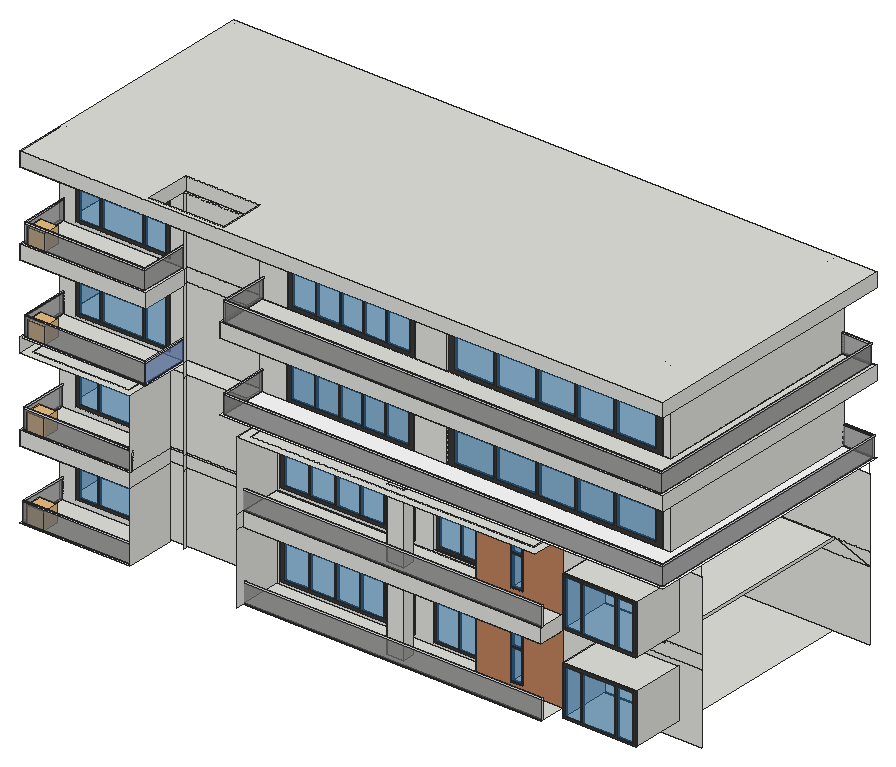
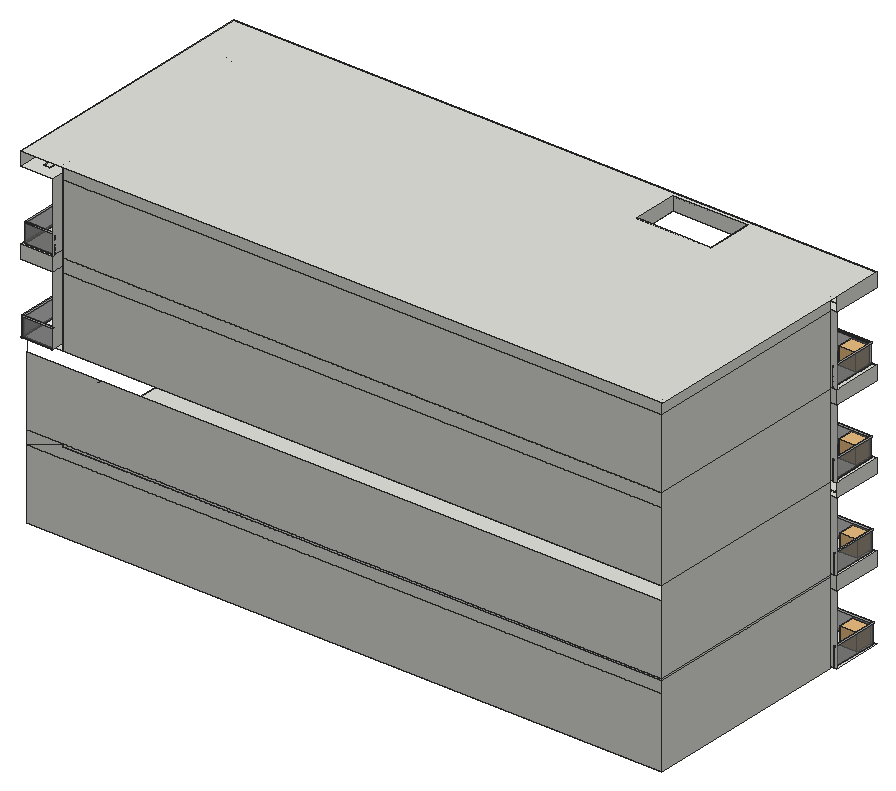
# SketchUp Ruby script. Lengths in inches.
U = 1.inch
M = Sketchup.active_model
def pt(a) = Geom::Point3d.new(a.map { |v| v * U })
def face(e, loops, mat)
  f = e.add_face(loops[0].map { |a| pt(a) })
  loops[1..].each { |l| e.add_face(l.map { |a| pt(a) }).erase! }
  f.material = f.back_material = mat if mat
  f
end
# faces: each face lists its corners as indices into pts; further lists are holes
def faces(e, pts, list, mat = nil) = list.each { |f| face(e, (f[0].is_a?(Array) ? f : [f]).map { |l| l.map { |i| pts[i] } }, mat) }
# xy, xz, yz: faces in a plane at the given z, y or x. An outline is a flat list of corners, or four numbers for a rectangle; further outlines are holes
def ring(l) = l.size == 4 ? [[l[0], l[1]], [l[2], l[1]], [l[2], l[3]], [l[0], l[3]]] : l.each_slice(2).to_a
def flat(e, list, mat, &to3) = list.each { |f| face(e, (f[0].is_a?(Array) ? f : [f]).map { |l| ring(l).map { |u, v| to3.(u, v) } }, mat) }
def xy(e, z, list, mat = nil) = flat(e, list, mat) { |x, y| [x, y, z] }
def xz(e, y, list, mat = nil) = flat(e, list, mat) { |x, z| [x, y, z] }
def yz(e, x, list, mat = nil) = flat(e, list, mat) { |y, z| [x, y, z] }
def lines(e, pts, list) = list.each { |a, b| e.add_line(pt(pts[a]), pt(pts[b])) }
# prism: a flat outline (further loops are holes) pulled along v
def prism(e, loops, v, mat = nil)
  f = face(e, loops, mat); d = Geom::Vector3d.new(v.map { |x| x * U })
  f.pushpull(f.normal.samedirection?(d) ? d.length : -d.length)
end
def box(e, o, s, mat = nil) = prism(e, [[o, [o[0] + s[0], o[1], o[2]], [o[0] + s[0], o[1] + s[1], o[2]], [o[0], o[1] + s[1], o[2]]]], [0, 0, s[2]], mat)
def at(x, y, z, deg = 0) = Geom::Transformation.translation(pt([x, y, z])) * Geom::Transformation.rotation(ORIGIN, Z_AXIS, deg.degrees)
def axes(o, x, y, z) = Geom::Transformation.new([*x, 0, *y, 0, *z, 0, *pt(o).to_a, 1])
def part(name) = M.definitions.add(name)
# library, detail: a bought-in or finely detailed component or shape, given as its bounding box
def library(name, o, s) = part(name).tap { |d| box(d.entities, o, s) }
def detail(e, o, s) = box(e.add_group.entities, o, s)
def put(e, d, t, mat = nil) = e.add_instance(d, t).tap { |i| i.material = mat if mat }
def group(e, t, mat = nil) = e.add_group.tap { |g| g.transformation = t; g.material = mat if mat }.entities
root = M.entities
M.materials.add("[Color M00]").color = [255, 255, 255]
M.materials.add("[Color M07]").color = [58, 58, 58]
M.materials.add("[Metal Silver]").color = [234, 233, 238]
M.materials.add("[Translucent Glass Blue]").color = [100, 149, 237]
M.materials["[Translucent Glass Blue]"].alpha = 0.5
M.materials.add("[Translucent Glass Gray]").color = [40, 128, 199]
M.materials["[Translucent Glass Gray]"].alpha = 0.5
M.materials.add("[Translucent Glass Gray]1").color = [128, 128, 128]
M.materials["[Translucent Glass Gray]1"].alpha = 0.5
M.materials.add("[Wood Veneer 02]").color = [190, 128, 91]
c1 = library("plants",[-16.3,-15.81,0],[32.6,31.62,37.8])
c2 = part("Group\#3")
xy(c2.entities,0,[[0,0,103.1875,6]],"[Color M07]")
xy(c2.entities,6.75,[[6.75,0,49.1,6],[51.71,0,96.4375,6]],"[Color M07]")
xy(c2.entities,160.21,[[6.75,0,49.1,6],[51.71,0,96.4375,6]],"[Color M07]")
xy(c2.entities,166.96,[[0,0,103.1875,6]],"[Color M07]")
xz(c2.entities,0,[[[0,0,103.1875,166.96],[51.71,6.75,96.4375,160.21],[6.75,6.75,49.1,160.21]]],"[Color M07]")
xz(c2.entities,0,[[6.75,6.75,49.1,160.21],[51.71,6.75,96.4375,160.21]],"[Translucent Glass Gray]")
xz(c2.entities,6,[[[0,0,103.1875,166.96],[51.71,6.75,96.4375,160.21],[6.75,6.75,49.1,160.21]]],"[Color M07]")
yz(c2.entities,0,[[0,0,6,166.96]],"[Color M07]")
yz(c2.entities,6.75,[[0,6.75,6,160.21]],"[Color M07]")
yz(c2.entities,49.1,[[0,6.75,6,160.21]],"[Color M07]")
yz(c2.entities,51.71,[[0,6.75,6,160.21]],"[Color M07]")
yz(c2.entities,96.4375,[[0,6.75,6,160.21]],"[Color M07]")
yz(c2.entities,103.1875,[[0,0,6,166.96]],"[Color M07]")
c3 = part("Group\#2")
xy(c3.entities,0,[[0,0,266.875,6]],"[Color M07]")
xy(c3.entities,9.27,[[9.27,0,57.67,6],[61.37,0,109.48,6],[113.18,0,157.6,6],[161.3,0,205.85,6],[209.55,0,257.6,6]],"[Color M07]")
xy(c3.entities,155.66,[[9.27,0,57.67,6],[61.37,0,109.48,6],[113.18,0,157.6,6],[161.3,0,205.85,6],[209.55,0,257.6,6]],"[Color M07]")
xy(c3.entities,164.9375,[[0,0,266.875,6]],"[Color M07]")
xz(c3.entities,0,[[[0,0,266.875,164.9375],[9.27,9.27,57.67,155.66],[61.37,9.27,109.48,155.66],[209.55,9.27,257.6,155.66],[161.3,9.27,205.85,155.66],[113.18,9.27,157.6,155.66]]],"[Color M07]")
xz(c3.entities,0,[[9.27,9.27,57.67,155.66],[61.37,9.27,109.48,155.66],[113.18,9.27,157.6,155.66],[161.3,9.27,205.85,155.66],[209.55,9.27,257.6,155.66]],"[Translucent Glass Gray]")
xz(c3.entities,6,[[[0,0,266.875,164.9375],[9.27,9.27,57.67,155.66],[61.37,9.27,109.48,155.66],[209.55,9.27,257.6,155.66],[161.3,9.27,205.85,155.66],[113.18,9.27,157.6,155.66]]],"[Color M07]")
yz(c3.entities,0,[[0,0,6,164.9375]],"[Color M07]")
yz(c3.entities,9.27,[[0,9.27,6,155.66]],"[Color M07]")
yz(c3.entities,57.67,[[0,9.27,6,155.66]],"[Color M07]")
yz(c3.entities,61.37,[[0,9.27,6,155.66]],"[Color M07]")
yz(c3.entities,109.48,[[0,9.27,6,155.66]],"[Color M07]")
yz(c3.entities,113.18,[[0,9.27,6,155.66]],"[Color M07]")
yz(c3.entities,157.6,[[0,9.27,6,155.66]],"[Color M07]")
yz(c3.entities,161.3,[[0,9.27,6,155.66]],"[Color M07]")
yz(c3.entities,205.85,[[0,9.27,6,155.66]],"[Color M07]")
yz(c3.entities,209.55,[[0,9.27,6,155.66]],"[Color M07]")
yz(c3.entities,257.6,[[0,9.27,6,155.66]],"[Color M07]")
yz(c3.entities,266.875,[[0,0,6,164.9375]],"[Color M07]")
c4 = part("Group\#4")
xy(c4.entities,0,[[0,0,117.92,3.42]],"[Color M07]")
xy(c4.entities,5.06,[[5.06,0,29.89,3.42],[33.27,0,84.5,3.42],[87.88,0,112.86,3.42]],"[Color M07]")
xy(c4.entities,112.86,[[5.06,0,29.89,3.42],[33.27,0,84.5,3.42],[87.88,0,112.86,3.42]],"[Color M07]")
xy(c4.entities,117.92,[[0,0,117.92,3.42]],"[Color M07]")
xz(c4.entities,0,[[[0,0,117.92,117.92],[33.27,5.06,84.5,112.86],[87.88,5.06,112.86,112.86],[5.06,5.06,29.89,112.86]]],"[Color M07]")
xz(c4.entities,0,[[5.06,5.06,29.89,112.86],[33.27,5.06,84.5,112.86],[87.88,5.06,112.86,112.86]],"[Translucent Glass Gray]")
xz(c4.entities,3.42,[[[0,0,117.92,117.92],[33.27,5.06,84.5,112.86],[87.88,5.06,112.86,112.86],[5.06,5.06,29.89,112.86]]],"[Color M07]")
yz(c4.entities,0,[[0,0,3.42,117.92]],"[Color M07]")
yz(c4.entities,5.06,[[0,5.06,3.42,112.86]],"[Color M07]")
yz(c4.entities,29.89,[[0,5.06,3.42,112.86]],"[Color M07]")
yz(c4.entities,33.27,[[0,5.06,3.42,112.86]],"[Color M07]")
yz(c4.entities,84.5,[[0,5.06,3.42,112.86]],"[Color M07]")
yz(c4.entities,87.88,[[0,5.06,3.42,112.86]],"[Color M07]")
yz(c4.entities,112.86,[[0,5.06,3.42,112.86]],"[Color M07]")
yz(c4.entities,117.92,[[0,0,3.42,117.92]],"[Color M07]")
c5 = part("Group\#5")
xy(c5.entities,0,[[0,0,33.625,2.4375]],"[Color M07]")
xy(c5.entities,2.77,[[2.77,0,30.85,2.4375]],"[Color M07]")
xy(c5.entities,92.73,[[2.77,0,30.85,2.4375]],"[Color M07]")
xy(c5.entities,95.66,[[2.77,0,30.85,2.4375]],"[Color M07]")
xy(c5.entities,164.1,[[2.77,0,30.85,2.4375]],"[Color M07]")
xy(c5.entities,166.875,[[0,0,33.625,2.4375]],"[Color M07]")
xz(c5.entities,0,[[[0,0,33.625,166.875],[2.77,2.77,30.85,92.73],[2.77,95.66,30.85,164.1]]],"[Color M07]")
xz(c5.entities,0,[[2.77,2.77,30.85,92.73],[2.77,95.66,30.85,164.1]],"[Translucent Glass Gray]")
xz(c5.entities,2.4375,[[[0,0,33.625,166.875],[2.77,2.77,30.85,92.73],[2.77,95.66,30.85,164.1]]],"[Color M07]")
yz(c5.entities,0,[[0,0,2.4375,166.875]],"[Color M07]")
yz(c5.entities,2.77,[[0,2.77,2.4375,92.73],[0,95.66,2.4375,164.1]],"[Color M07]")
yz(c5.entities,30.85,[[0,2.77,2.4375,92.73],[0,95.66,2.4375,164.1]],"[Color M07]")
yz(c5.entities,33.625,[[0,0,2.4375,166.875]],"[Color M07]")
xy(root,585,[[0,191.16,284.54,191.16,284.54,195.23,3.5,195.23,3.5,320.73,0,320.73],[3.5,195.23,3.5,320.73,5.5,320.73,5.5,197.23,284.54,197.23,284.54,195.23],[5.5,197.23,284.54,320.73],[559.99,210.66,1334.26,213.98],[559.99,213.98,1334.26,215.98],
  [[559.99,215.98,1334.26,215.98,1334.26,280.1,1109.39,280.1,1109.39,320.73,559.99,320.73],[917.6,232.38,960.55,263.125]],[917.6,232.38,960.55,263.125],[1109.39,280.1,1334.26,320.73],[9.75,328.54,1561.7,873.45]])
xy(root,589.69,[[967.92,320.73,1101.04,328.54]])
xy(root,590.74,[[568.97,320.73,917.6,328.54]])
xy(root,596.29,[[40.45,320.73,260.7,328.54]])
xy(root,599.96,[[1200.375,280.1,1230.875,328.54]])
xy(root,625.17,[[1405.04,191.16,1595.91,328.54]])
xy(root,633,[[3.5,195.23,3.5,320.73,5.5,320.73,5.5,197.23,284.54,197.23,284.54,195.23],[559.99,213.98,1334.26,215.98]],"[Metal Silver]")
xy(root,637,[[3.5,195.23,284.54,195.23,284.54,197.23,5.5,197.23,5.5,320.73,3.5,320.73],[559.99,213.98,1334.26,215.98]],"[Metal Silver]")
xy(root,733.42,[[568.97,320.73,917.6,328.54],[967.92,320.73,1101.04,328.54]])
xy(root,746.15,[[1200.375,280.1,1230.875,328.54]])
xy(root,750.17,[[40.45,320.73,260.7,328.54]])
xy(root,753.48,[[1405.04,191.16,1595.91,328.54]])
xy(root,757,[[[578.25,228.93,578.25,302.47,1091.125,302.47,1091.125,261.84,1316,261.84,1316,228.93],[917.6,232.38,960.55,263.125]]])
xy(root,760,[[20.05,211.22,264.48,300.67]])
xy(root,765,[[[0,191.16,284.54,320.73],[20.05,211.22,264.48,300.67]],[[559.99,210.66,559.99,320.73,1109.39,320.73,1109.39,280.1,1334.26,280.1,1334.26,210.66],[578.25,228.93,1316,228.93,1316,261.84,1091.125,261.84,1091.125,302.47,578.25,302.47]],[20.05,211.22,264.48,300.67],[[578.25,228.93,1316,228.93,1316,261.84,1091.125,261.84,1091.125,302.47,578.25,302.47],[917.6,232.38,960.55,263.125]],[917.6,232.38,960.55,263.125],
  [1109.39,280.1,1334.26,320.73]])
xy(root,795,[[9.75,328.54,1561.7,873.45]])
xy(root,801,[[0,191.16,284.54,191.16,284.54,196.41,4.5,196.41,4.5,320.73,0,320.73],[4.5,196.41,4.5,320.73,6.5,320.73,6.5,198.41,284.54,198.41,284.54,196.41],[6.5,198.41,284.54,320.73],[559.99,210.66,1334.26,213.16],[559.99,213.16,1334.26,215.16],
  [[559.99,215.16,1334.26,215.16,1334.26,280.1,1109.39,280.1,1109.39,320.73,559.99,320.73],[917.6,232.38,960.55,263.125]],[917.6,232.38,960.55,263.125],[1109.39,280.1,1334.26,320.73],[9.75,328.54,1561.7,873.45]])
xy(root,805.07,[[967.92,320.73,1101.04,328.54]])
xy(root,808.99,[[568.97,320.73,917.6,328.54]])
xy(root,812.92,[[40.45,320.73,260.7,328.54]])
xy(root,818.15,[[1200.375,280.1,1230.875,328.54]])
xy(root,832.73,[[1405.04,191.16,1595.91,328.54]])
xy(root,849,[[4.5,196.41,4.5,320.73,6.5,320.73,6.5,198.41,284.54,198.41,284.54,196.41],[559.99,213.16,1334.26,215.16]],"[Metal Silver]")
xy(root,853,[[4.5,196.41,284.54,196.41,284.54,198.41,6.5,198.41,6.5,320.73,4.5,320.73],[559.99,213.16,1334.26,215.16]],"[Metal Silver]")
xy(root,958.6,[[568.97,320.73,917.6,328.54],[967.92,320.73,1101.04,328.54]])
xy(root,961.04,[[1405.04,191.16,1595.91,328.54]])
xy(root,964.33,[[1200.375,280.1,1230.875,328.54]])
xy(root,966.79,[[40.45,320.73,260.7,328.54]])
xy(root,973,[[[581.03,212.21,581.03,299.68,1088.34,299.68,1088.34,259.06,1313.21,259.06,1313.21,212.21],[917.6,232.38,960.55,263.125]]])
xy(root,976,[[17.39,208.55,267.15,303.34]])
xy(root,981,[[[0,191.16,284.54,320.73],[17.39,208.55,267.15,303.34]],[[559.99,191.16,559.99,320.73,1109.39,320.73,1109.39,280.1,1334.26,280.1,1334.26,191.16],[581.03,212.21,1313.21,212.21,1313.21,259.06,1088.34,259.06,1088.34,299.68,581.03,299.68]],[17.39,208.55,267.15,303.34],[[581.03,212.21,1313.21,212.21,1313.21,259.06,1088.34,259.06,1088.34,299.68,581.03,299.68],[917.6,232.38,960.55,263.125]],[917.6,232.38,960.55,263.125]])
xy(root,1017,[[0,191.16,324.77,191.16,324.77,320.73,320.15,320.73,320.15,196.41,6.6875,196.41,6.6875,320.73,0,320.73],[6.6875,196.41,6.6875,320.73,8.6875,320.73,8.6875,198.41,318.15,198.41,318.15,320.73,320.15,320.73,320.15,196.41],[8.6875,198.41,318.15,320.73],[587.47,320.73,915.35,328.54],[915.35,320.73,1002.83,328.54],
  [1002.83,320.73,1561.7,328.54],[1561.7,320.73,1581.35,328.54],[9.75,328.54,1561.7,873.45],[1561.7,328.54,1581.35,873.45]])
xy(root,1017,[[518.01,191.16,518.01,320.73,523.33,320.73,523.33,196.23,1661.42,196.23,1661.42,882.43,1665.48,882.45,1665.48,191.16],[525.33,198.23,525.33,320.73,1581.35,320.73,1581.35,879.63,1659.42,879.63,1659.42,198.23],[1581.35,879.63,1581.35,881.99,1659.42,882.42,1659.42,879.63],[1581.35,881.99,1659.42,882.42,1659.42,882.45,1581.35,882.45],[1659.42,882.42,1661.42,882.43,1661.42,882.45,1659.42,882.45],
  [1661.42,882.43,1665.48,882.45,1661.42,882.45]],"[Color M00]")
xy(root,1017,[[523.33,196.23,523.33,320.73,525.33,320.73,525.33,198.23,1659.42,198.23,1659.42,882.42,1661.42,882.43,1661.42,196.23]],"[Translucent Glass Gray]1")
xy(root,1024.1,[[41.07,320.73,283.01,328.54]])
xy(root,1065,[[523.33,196.23,523.33,320.73,525.33,320.73,525.33,198.23,1659.42,198.23,1659.42,882.42,1661.42,882.43,1661.42,196.23],[6.6875,196.41,6.6875,320.73,8.6875,320.73,8.6875,198.41,318.15,198.41,318.15,320.73,320.15,320.73,320.15,196.41],[1581.35,879.63,1581.35,881.99,1659.42,882.42,1659.42,879.63]],"[Metal Silver]")
xy(root,1069,[[523.33,196.23,1661.42,196.23,1661.42,882.43,1581.35,881.99,1581.35,879.63,1659.42,879.63,1659.42,198.23,525.33,198.23,525.33,320.73,523.33,320.73],[6.6875,196.41,320.15,196.41,320.15,320.73,318.15,320.73,318.15,198.41,8.6875,198.41,8.6875,320.73,6.6875,320.73]],"[Metal Silver]")
xy(root,1160.71,[[587.47,320.73,915.35,328.54],[1002.83,320.73,1561.7,328.54]])
xy(root,1187.47,[[41.07,320.73,283.01,328.54]])
xy(root,1189,[[552.125,216.56,552.125,295.33,1606.75,295.33,1606.75,857.05,1640.08,857.05,1640.08,216.56]])
xy(root,1197,[[[0,191.16,324.77,320.73],[20.91,212.07,303.87,299.82]],[[518.01,191.16,518.01,320.73,1581.35,320.73,1581.35,882.45,1665.48,882.45,1665.48,191.16],[552.125,216.56,1640.08,216.56,1640.08,857.05,1606.75,857.05,1606.75,295.33,552.125,295.33]],[20.91,212.07,303.87,299.82],[552.125,216.56,1640.08,216.56,1640.08,857.05,1606.75,857.05,1606.75,295.33,552.125,295.33]])
xy(root,1233,[[0,191.16,324.77,191.16,324.77,320.73,319.34,320.73,319.34,196.04,8.125,196.04,8.125,320.73,0,320.73],[518.01,191.16,1665.48,191.16,1665.48,882.45,1581.35,882.45,1581.35,877.14,1658.85,877.14,1658.85,195.23,524.95,195.23,524.95,320.73,518.01,320.73],[524.95,195.23,524.95,320.73,526.95,320.73,526.95,197.23,1656.85,197.23,1656.85,875.14,1658.85,875.14,1658.85,195.23],[8.125,196.04,8.125,320.73,10.125,320.73,10.125,198.04,317.34,198.04,317.34,320.73,319.34,320.73,319.34,196.04],[526.95,197.23,1656.85,197.23,1656.85,875.14,1581.35,875.14,1581.35,320.73,526.95,320.73],
  [10.125,198.04,317.34,320.73],[590.16,320.73,918.03,328.54],[1002.83,320.73,1561.7,328.54],[9.75,328.54,1561.7,873.45]])
xy(root,1241.47,[[41.07,320.73,283.01,328.54]])
xy(root,1281,[[524.95,195.23,524.95,320.73,526.95,320.73,526.95,197.23,1656.85,197.23,1656.85,875.14,1658.85,875.14,1658.85,195.23],[8.125,196.04,8.125,320.73,10.125,320.73,10.125,198.04,317.34,198.04,317.34,320.73,319.34,320.73,319.34,196.04],[1581.35,875.14,1658.85,877.14]],"[Metal Silver]")
xy(root,1285,[[524.95,195.23,1658.85,195.23,1658.85,877.14,1581.35,877.14,1581.35,875.14,1656.85,875.14,1656.85,197.23,526.95,197.23,526.95,320.73,524.95,320.73],[8.125,196.04,319.34,196.04,319.34,320.73,317.34,320.73,317.34,198.04,10.125,198.04,10.125,320.73,8.125,320.73]],"[Metal Silver]")
xy(root,1383.58,[[590.16,320.73,918.03,328.54],[1002.83,320.73,1561.7,328.54]])
xy(root,1404.85,[[41.07,320.73,283.01,328.54]])
xy(root,1405,[[24.96,217.75,297.46,291.5625],[552.125,225.28,552.125,286.62,1615.47,286.62,1615.47,848.34,1631.37,848.34,1631.37,225.28]])
xy(root,1413,[[[0,191.16,0,320.73,324.77,320.73,324.77,202.74,518.01,202.74,518.01,191.16],[24.96,217.75,297.46,291.5625]],[[518.01,191.16,518.01,320.73,1581.35,320.73,1581.35,882.45,1665.48,882.45,1665.48,191.16],[552.125,225.28,1631.37,225.28,1631.37,848.34,1615.47,848.34,1615.47,286.62,552.125,286.62]],[24.96,217.75,297.46,291.5625],[552.125,225.28,1631.37,225.28,1631.37,848.34,1615.47,848.34,1615.47,286.62,552.125,286.62],[324.77,313.48,334,320.73],
  [341.5,313.48,349,320.73],[356.5,313.48,364,320.73],[371.5,313.48,379,320.73],[386.5,313.48,394,320.73],[401.5,313.48,409,320.73],
  [416.5,313.48,424,320.73],[431.5,313.48,439,320.73],[446.5,313.48,454,320.73],[461.5,313.48,469,320.73],[476.5,313.48,484,320.73],
  [491.5,313.48,499,320.73],[506.5,313.48,514,320.73]])
xy(root,1443,[[9.75,328.54,1561.7,873.45]])
xy(root,1449,[[[0,191.16,1665.48,882.45],[324.77,202.74,518.01,320.73]]])
xz(root,191.16,[[0,765,284.54,801],[0,1197,324.77,1233],[518.01,1197,1665.48,1233],[0,1413,1665.48,1449]])
xz(root,195.23,[[3.5,633,284.54,637],[524.95,1281,1658.85,1285]],"[Metal Silver]")
xz(root,195.23,[[3.5,585,284.54,633],[524.95,1233,1658.85,1281]],"[Translucent Glass Gray]1")
xz(root,196.04,[[8.125,1281,319.34,1285]],"[Metal Silver]")
xz(root,196.04,[[8.125,1233,319.34,1281]],"[Translucent Glass Gray]1")
xz(root,196.23,[[523.33,1065,1661.42,1069]],"[Metal Silver]")
xz(root,196.23,[[523.33,1017,1661.42,1065]],"[Translucent Glass Gray]1")
xz(root,196.41,[[4.5,849,284.54,853],[6.6875,1065,320.15,1069]],"[Metal Silver]")
xz(root,196.41,[[4.5,801,284.54,849],[6.6875,1017,320.15,1065]],"[Translucent Glass Gray]1")
xz(root,197.23,[[5.5,633,284.54,637],[526.95,1281,1656.85,1285]],"[Metal Silver]")
xz(root,197.23,[[5.5,585,284.54,633],[526.95,1233,1656.85,1281]],"[Translucent Glass Gray]1")
xz(root,198.04,[[10.125,1281,317.34,1285]],"[Metal Silver]")
xz(root,198.04,[[10.125,1233,317.34,1281]],"[Translucent Glass Gray]1")
xz(root,198.23,[[525.33,1065,1659.42,1069]],"[Metal Silver]")
xz(root,198.23,[[525.33,1017,1659.42,1065]],"[Translucent Glass Gray]1")
xz(root,198.41,[[6.5,849,284.54,853],[8.6875,1065,318.15,1069]],"[Metal Silver]")
xz(root,198.41,[[6.5,801,284.54,849],[8.6875,1017,318.15,1065]],"[Translucent Glass Gray]1")
xz(root,202.74,[[324.77,1413,518.01,1449]])
xz(root,208.55,[[17.39,976,267.15,981]])
xz(root,210.66,[[559.99,765,1334.26,801]])
xz(root,211.22,[[20.05,760,264.48,765]])
xz(root,212.21,[[581.03,973,1313.21,981]])
xz(root,213.16,[[559.99,849,1334.26,853]],"[Metal Silver]")
xz(root,213.16,[[559.99,801,1334.26,849]],"[Translucent Glass Gray]1")
xz(root,213.98,[[559.99,633,1334.26,637]],"[Metal Silver]")
xz(root,213.98,[[559.99,585,1334.26,633]],"[Translucent Glass Gray]1")
xz(root,215.16,[[559.99,849,1334.26,853]],"[Metal Silver]")
xz(root,215.16,[[559.99,801,1334.26,849]],"[Translucent Glass Gray]1")
xz(root,215.98,[[559.99,633,1334.26,637]],"[Metal Silver]")
xz(root,215.98,[[559.99,585,1334.26,633]],"[Translucent Glass Gray]1")
xz(root,216.56,[[552.125,1189,1640.08,1197]])
xz(root,217.75,[[24.96,1405,297.46,1413]])
xz(root,225.28,[[552.125,1405,1631.37,1413]])
xz(root,228.93,[[578.25,757,1316,765]])
xz(root,232.38,[[917.6,585,960.55,757],[917.6,757,960.55,765],[917.6,801,960.55,973],[917.6,973,960.55,981]])
xz(root,259.06,[[1088.34,973,1313.21,981]])
xz(root,261.84,[[1091.125,757,1316,765]])
xz(root,263.125,[[917.6,585,960.55,757],[917.6,757,960.55,765],[917.6,801,960.55,973],[917.6,973,960.55,981]])
xz(root,280.1,[[[1109.39,585,1334.26,765],[1200.375,599.96,1230.875,746.15]],[[1109.39,801,1334.26,981],[1200.375,818.15,1230.875,964.33]]],"[Wood Veneer 02]")
xz(root,286.62,[[552.125,1405,1615.47,1413]])
xz(root,291.5625,[[24.96,1405,297.46,1413]])
xz(root,295.33,[[552.125,1189,1606.75,1197]])
xz(root,299.68,[[581.03,973,1088.34,981]])
xz(root,300.67,[[20.05,760,264.48,765]])
xz(root,302.47,[[578.25,757,917.6,765],[917.6,757,960.55,765],[960.55,757,1091.125,765]])
xz(root,303.34,[[17.39,976,267.15,981]])
xz(root,320.73,[[[0,585,3.5,585,3.5,637,5.5,637,5.5,585,284.54,585,284.54,765,0,765],[40.45,596.29,260.7,750.17]],[3.5,585,5.5,633],[[559.99,585,1109.39,765],[568.97,590.74,917.6,733.42],[967.92,589.69,1101.04,733.42]],[0,765,284.54,801],[559.99,765,917.6,801],
  [917.6,765,960.55,801],[960.55,765,1109.39,801],[1109.39,765,1334.26,801],[[0,801,4.5,801,4.5,853,6.5,853,6.5,801,284.54,801,284.54,981,0,981],[40.45,812.92,260.7,966.79]],[4.5,801,6.5,849],
  [[559.99,801,1109.39,981],[568.97,808.99,917.6,958.6],[967.92,805.07,1101.04,958.6]],[[0,1017,6.6875,1017,6.6875,1069,8.6875,1069,8.6875,1017,318.15,1017,318.15,1069,320.15,1069,320.15,1017,324.77,1017,324.77,1197,0,1197],[41.07,1024.1,283.01,1187.47]],[6.6875,1017,8.6875,1065],[318.15,1017,320.15,1065],[518.01,1017,523.33,1017,523.33,1069,525.33,1069,525.33,1017,587.47,1017,587.47,1160.71,915.35,1160.71,915.35,1017,1002.83,1017,1002.83,1160.71,1561.7,1160.71,1561.7,1017,1581.35,1017,1581.35,1197,518.01,1197],
  [0,1197,324.77,1233],[518.01,1197,521.5,1233],[521.5,1197,529,1233],[529,1197,536.5,1233],[536.5,1197,1581.35,1233],
  [[0,1233,8.125,1233,8.125,1285,10.125,1285,10.125,1233,317.34,1233,317.34,1285,319.34,1285,319.34,1233,324.77,1233,324.77,1413,0,1413],[41.07,1241.47,283.01,1404.85]],[8.125,1233,10.125,1281],[317.34,1233,319.34,1281],[518.01,1233,524.95,1233,524.95,1285,526.95,1285,526.95,1233,590.16,1233,590.16,1383.58,918.03,1383.58,918.03,1233,1002.83,1233,1002.83,1383.58,1561.7,1383.58,1561.7,1233,1581.35,1233,1581.35,1413,518.01,1413],[524.95,1233,526.95,1281],
  [324.77,1413,518.01,1449]])
xz(root,320.73,[[3.5,633,5.5,637],[4.5,849,6.5,853],[6.6875,1065,8.6875,1069],[318.15,1065,320.15,1069],[523.33,1065,525.33,1069],
  [8.125,1281,10.125,1285],[317.34,1281,319.34,1285],[524.95,1281,526.95,1285]],"[Metal Silver]")
xz(root,320.73,[[523.33,1017,525.33,1065]],"[Translucent Glass Gray]1")
xz(root,328.54,[[[9.75,585,1655.73,765],[568.97,590.74,917.6,733.42],[40.45,596.29,260.7,750.17],[1405.04,625.17,1595.91,753.48],[967.92,589.69,1101.04,733.42],[1200.375,599.96,1230.875,746.15]],[9.75,765,9.75,795,1561.7,795,1561.7,801,1655.73,801,1655.73,765],[9.75,795,1561.7,801],[[9.75,801,1655.73,981],[568.97,808.99,917.6,958.6],[40.45,812.92,260.7,966.79],[1405.04,832.73,1595.91,961.04],[967.92,805.07,1101.04,958.6],[1200.375,818.15,1230.875,964.33]],[[9.75,1017,9.75,1197,1561.7,1197,1561.7,1160.71,1002.83,1160.71,1002.83,1017,915.35,1017,915.35,1160.71,587.47,1160.71,587.47,1017],[41.07,1024.1,283.01,1187.47]],
  [587.47,1017,915.35,1160.71],[1002.83,1017,1561.7,1160.71],[9.75,1197,1561.7,1233],[[9.75,1233,9.75,1413,1561.7,1413,1561.7,1383.58,1002.83,1383.58,1002.83,1233,918.03,1233,918.03,1383.58,590.16,1383.58,590.16,1233],[41.07,1241.47,283.01,1404.85]],[9.75,1413,1561.7,1443]])
xz(root,848.34,[[1615.47,1405,1631.37,1413]])
xz(root,857.05,[[1606.75,1189,1640.08,1197]])
xz(root,873.45,[[9.75,585,1655.73,765],[9.75,765,1655.73,765,1561.7,801,1561.7,795,9.75,795],[1655.73,765,1655.73,801,1561.7,801],[9.75,795,1561.7,801],[9.75,801,1655.73,981],
  [9.75,1017,1561.7,1197],[9.75,1197,1561.7,1233],[9.75,1233,1561.7,1413],[9.75,1413,1561.7,1443]])
xz(root,875.14,[[1581.35,1281,1656.85,1285]],"[Metal Silver]")
xz(root,875.14,[[1581.35,1233,1656.85,1281]],"[Translucent Glass Gray]1")
xz(root,877.14,[[1581.35,1281,1658.85,1285]],"[Metal Silver]")
xz(root,877.14,[[1581.35,1233,1658.85,1281]],"[Translucent Glass Gray]1")
xz(root,879.63,[[1581.35,1065,1659.42,1069]],"[Metal Silver]")
xz(root,879.63,[[1581.35,1017,1659.42,1065]],"[Translucent Glass Gray]1")
xz(root,882.45,[[1581.35,1197,1665.48,1233]])
yz(root,0,[[191.16,765,320.73,801],[191.16,981,320.73,1017],[191.16,1197,320.73,1233],[191.16,1413,320.73,1449]])
yz(root,3.5,[[195.23,633,320.73,637]],"[Metal Silver]")
yz(root,3.5,[[195.23,585,320.73,633]],"[Translucent Glass Gray]1")
yz(root,4.5,[[196.41,849,320.73,853]],"[Metal Silver]")
yz(root,4.5,[[196.41,801,320.73,849]],"[Translucent Glass Gray]1")
yz(root,5.5,[[197.23,633,320.73,637]],"[Metal Silver]")
yz(root,5.5,[[197.23,585,320.73,633]],"[Translucent Glass Gray]1")
yz(root,6.5,[[198.41,849,320.73,853]],"[Metal Silver]")
yz(root,6.5,[[198.41,801,320.73,849]],"[Translucent Glass Gray]1")
yz(root,6.6875,[[196.41,1065,320.73,1069]],"[Metal Silver]")
yz(root,6.6875,[[196.41,1017,320.73,1065]],"[Translucent Glass Gray]1")
yz(root,8.125,[[196.04,1281,320.73,1285]],"[Metal Silver]")
yz(root,8.125,[[196.04,1233,320.73,1281]],"[Translucent Glass Gray]1")
yz(root,8.6875,[[198.41,1065,320.73,1069]],"[Metal Silver]")
yz(root,8.6875,[[198.41,1017,320.73,1065]],"[Translucent Glass Gray]1")
yz(root,9.75,[[328.54,585,873.45,795],[328.54,795,873.45,801],[328.54,801,873.45,1017],[328.54,1017,873.45,1233],[328.54,1233,873.45,1413],
  [328.54,1413,873.45,1443]])
yz(root,10.125,[[198.04,1281,320.73,1285]],"[Metal Silver]")
yz(root,10.125,[[198.04,1233,320.73,1281]],"[Translucent Glass Gray]1")
yz(root,17.39,[[208.55,976,303.34,981]])
yz(root,20.05,[[211.22,760,300.67,765]])
yz(root,24.96,[[217.75,1405,291.5625,1413]])
yz(root,40.45,[[320.73,596.29,328.54,750.17],[320.73,812.92,328.54,966.79]])
yz(root,41.07,[[320.73,1024.1,328.54,1187.47],[320.73,1241.47,328.54,1404.85]])
yz(root,260.7,[[320.73,596.29,328.54,750.17],[320.73,812.92,328.54,966.79]])
yz(root,264.48,[[211.22,760,300.67,765]])
yz(root,267.15,[[208.55,976,303.34,981]])
yz(root,283.01,[[320.73,1024.1,328.54,1187.47],[320.73,1241.47,328.54,1404.85]])
yz(root,284.54,[[191.16,585,191.16,765,320.73,765,320.73,585,197.23,585,197.23,637,195.23,637,195.23,585],[195.23,585,197.23,633],[191.16,765,320.73,801],[191.16,801,191.16,981,320.73,981,320.73,801,198.41,801,198.41,853,196.41,853,196.41,801],[196.41,801,198.41,849]])
yz(root,284.54,[[195.23,633,197.23,637],[196.41,849,198.41,853]],"[Metal Silver]")
yz(root,297.46,[[217.75,1405,291.5625,1413]])
yz(root,317.34,[[198.04,1281,320.73,1285]],"[Metal Silver]")
yz(root,317.34,[[198.04,1233,320.73,1281]],"[Translucent Glass Gray]1")
yz(root,318.15,[[198.41,1065,320.73,1069]],"[Metal Silver]")
yz(root,318.15,[[198.41,1017,320.73,1065]],"[Translucent Glass Gray]1")
yz(root,319.34,[[196.04,1281,320.73,1285]],"[Metal Silver]")
yz(root,319.34,[[196.04,1233,320.73,1281]],"[Translucent Glass Gray]1")
yz(root,320.15,[[196.41,1065,320.73,1069]],"[Metal Silver]")
yz(root,320.15,[[196.41,1017,320.73,1065]],"[Translucent Glass Blue]")
yz(root,324.77,[[313.48,585,320.73,765],[313.48,765,320.73,801],[313.48,801,320.73,981],[313.48,981,320.73,1017],[313.48,1017,320.73,1197],
  [191.16,1197,313.48,1233],[313.48,1197,320.73,1233],[313.48,1233,320.73,1413],[202.74,1413,320.73,1449]])
yz(root,518.01,[[191.16,1197,320.73,1233],[202.74,1413,320.73,1449]])
yz(root,523.33,[[196.23,1065,320.73,1069]],"[Metal Silver]")
yz(root,523.33,[[196.23,1017,320.73,1065]],"[Translucent Glass Gray]1")
yz(root,524.95,[[195.23,1281,320.73,1285]],"[Metal Silver]")
yz(root,524.95,[[195.23,1233,320.73,1281]],"[Translucent Glass Gray]1")
yz(root,525.33,[[198.23,1065,320.73,1069]],"[Metal Silver]")
yz(root,525.33,[[198.23,1017,320.73,1065]],"[Translucent Glass Gray]1")
yz(root,526.95,[[197.23,1281,320.73,1285]],"[Metal Silver]")
yz(root,526.95,[[197.23,1233,320.73,1281]],"[Translucent Glass Gray]1")
yz(root,552.125,[[216.56,1189,295.33,1197],[225.28,1405,286.62,1413]])
yz(root,559.99,[[191.16,585,213.98,585,213.98,637,215.98,637,215.98,585,320.73,585,320.73,765,191.16,765],[213.98,585,215.98,633],[191.16,765,210.66,801],[210.66,765,320.73,801],[191.16,801,213.16,801,213.16,853,215.16,853,215.16,801,320.73,801,320.73,981,191.16,981],
  [213.16,801,215.16,849]])
yz(root,559.99,[[213.98,633,215.98,637],[213.16,849,215.16,853]],"[Metal Silver]")
yz(root,568.97,[[320.73,590.74,328.54,733.42],[320.73,808.99,328.54,958.6]])
yz(root,578.25,[[228.93,757,302.47,765]])
yz(root,581.03,[[212.21,973,299.68,981]])
yz(root,587.47,[[320.73,1017,328.54,1160.71]])
yz(root,590.16,[[320.73,1233,328.54,1383.58]])
yz(root,915.35,[[320.73,1017,328.54,1160.71]])
yz(root,917.6,[[232.38,585,263.125,757],[320.73,590.74,328.54,733.42],[232.38,757,263.125,765],[232.38,801,263.125,973],[320.73,808.99,328.54,958.6],
  [232.38,973,263.125,981]])
yz(root,918.03,[[320.73,1233,328.54,1383.58]])
yz(root,960.55,[[232.38,585,263.125,757],[232.38,757,263.125,765],[232.38,801,263.125,973],[232.38,973,263.125,981]])
yz(root,967.92,[[320.73,589.69,328.54,733.42],[320.73,805.07,328.54,958.6]])
yz(root,1002.83,[[320.73,1017,328.54,1160.71],[320.73,1233,328.54,1383.58]])
yz(root,1088.34,[[259.06,973,299.68,981]])
yz(root,1091.125,[[261.84,757,302.47,765]])
yz(root,1101.04,[[320.73,589.69,328.54,733.42],[320.73,805.07,328.54,958.6]])
yz(root,1109.39,[[280.1,585,320.73,765],[280.1,801,320.73,981]],"[Wood Veneer 02]")
yz(root,1200.375,[[280.1,599.96,328.54,746.15],[280.1,818.15,328.54,964.33]])
yz(root,1230.875,[[280.1,599.96,328.54,746.15],[280.1,818.15,328.54,964.33]])
yz(root,1313.21,[[212.21,973,259.06,981]])
yz(root,1316,[[228.93,757,261.84,765]])
yz(root,1334.26,[[213.98,585,215.98,633],[210.66,765,320.73,801],[213.16,801,215.16,849]])
yz(root,1334.26,[[213.98,633,215.98,637],[213.16,849,215.16,853]],"[Metal Silver]")
yz(root,1405.04,[[191.16,625.17,328.54,753.48],[191.16,832.73,328.54,961.04]])
yz(root,1561.7,[[328.54,795,873.45,801],[320.73,1017,328.54,1160.71],[328.54,1017,873.45,1233],[320.73,1233,328.54,1383.58],[328.54,1233,873.45,1443]])
yz(root,1581.35,[[320.73,1017,879.63,1017,879.63,1069,881.99,1069,881.99,1017,882.45,1017,882.45,1197,320.73,1197],[320.73,1197,882.45,1197,882.45,1233,877.14,1233,877.14,1281,875.14,1281,875.14,1233,320.73,1233],[320.73,1233,875.14,1233,875.14,1285,877.14,1285,877.14,1233,882.45,1233,882.45,1413,320.73,1413]])
yz(root,1581.35,[[879.63,1017,881.99,1065]],"[Color M00]")
yz(root,1581.35,[[879.63,1065,881.99,1069],[875.14,1281,877.14,1285]],"[Metal Silver]")
yz(root,1595.91,[[191.16,625.17,328.54,753.48],[191.16,832.73,328.54,961.04]])
yz(root,1606.75,[[295.33,1189,857.05,1197]])
yz(root,1615.47,[[286.62,1405,848.34,1413]])
yz(root,1631.37,[[225.28,1405,848.34,1413]])
yz(root,1640.08,[[216.56,1189,857.05,1197]])
yz(root,1656.85,[[197.23,1281,875.14,1285]],"[Metal Silver]")
yz(root,1656.85,[[197.23,1233,875.14,1281]],"[Translucent Glass Gray]1")
yz(root,1658.85,[[195.23,1281,877.14,1285]],"[Metal Silver]")
yz(root,1658.85,[[195.23,1233,877.14,1281]],"[Translucent Glass Gray]1")
yz(root,1659.42,[[879.63,1017,882.42,1065]],"[Color M00]")
yz(root,1659.42,[[198.23,1065,879.63,1069]],"[Metal Silver]")
yz(root,1659.42,[[198.23,1017,879.63,1065]],"[Translucent Glass Gray]1")
yz(root,1661.42,[[196.23,1065,882.43,1069]],"[Metal Silver]")
yz(root,1661.42,[[196.23,1017,882.43,1065]],"[Translucent Glass Gray]1")
yz(root,1665.48,[[191.16,1197,882.45,1233],[191.16,1413,882.45,1449]])
p = [[1659.42,882.42,1017],[1581.35,881.99,1017],[1581.35,881.99,1065],[1659.42,882.42,1065],[1661.42,882.43,1017],[1661.42,882.43,1065],
  [1581.35,881.99,1069],[1661.42,882.43,1069],[1655.73,873.45,981],[1655.73,873.45,1017],[1581.35,320.73,1413],[1581.35,320.73,1449],
  [1655.73,328.54,981],[1655.73,328.54,1017],[1464.9,882.45,981],[1464.9,873.45,981],[1561.7,854.2,1449],[1561.7,854.2,1443],
  [9.75,328.54,1443],[9.75,328.54,1449],[9.75,873.45,1443],[9.75,873.45,1449],[1561.7,328.54,1443],[1561.7,328.54,1449],
  [1561.7,873.45,1443],[1561.7,873.45,1449]]
faces(root,p,[[0,1,2,3],[4,0,3,5]],"[Translucent Glass Gray]1")
faces(root,p,[[2,6,7,5,3]],"[Metal Silver]")
lines(root,p,[[8,9],[10,11],[12,13],[14,15],[16,17],[18,19],[20,21],[22,23],[24,25]])
put(root,c1,axes([34.4,218.09,585],[1.38,0,0],[0,1.32,0],[0,0,1.15]))
put(root,c2,axes([967.92,321.05,589.69],[1.29013,0,0],[0,0.49104,0],[0,0,0.85928]))
put(root,c3,axes([568.97,321.03,590.74],[1.30633,0,0],[0,0.7802,0],[0,0,0.86506]))
put(root,c4,axes([40.45,320.73,596.29],[1.86781,0,0],[0,1,0],[0,0,1.30492]))
put(root,c5,axes([1200.375,280.1,599.96],[0.90706,0,0],[0,2.4,0],[0,0,0.87603]))
put(root,c4,axes([1405.04,191.16,625.17],[1.6187,0,0],[0,1,0],[0,0,1.08814]))
put(root,c1,axes([34.08,217.28,801],[1.38,0,0],[0,1.32,0],[0,0,1.15]))
put(root,c2,axes([967.92,328.87,805.07],[1.29013,0,0],[0,0.49104,0],[0,0,0.9196]))
put(root,c3,axes([568.97,321.03,808.99],[1.30633,0,0],[0,0.7802,0],[0,0,0.90831]))
put(root,c4,axes([40.45,320.73,812.92],[1.86781,0,0],[0,1,0],[0,0,1.30492]))
put(root,c5,axes([1200.375,280.1,818.15],[0.90706,0,0],[0,2.4,0],[0,0,0.87603]))
put(root,c4,axes([1405.04,191.16,832.73],[1.6187,0,0],[0,1,0],[0,0,1.08814]))
put(root,c3,axes([1002.83,321.75,1017],[2.09415,0,0],[0,0.83,0],[0,0,0.87128]))
put(root,c3,axes([587.64,321.01,1017],[1.22795,0,0],[0,0.73339,0],[0,0,0.87128]))
put(root,c1,axes([37.94,217.28,1017],[1.38,0,0],[0,1.32,0],[0,0,1.15]))
put(root,c4,axes([41.07,320.73,1024.1],[2.05173,0,0],[0,1,0],[0,0,1.38549]))
put(root,c3,axes([1002.83,321.75,1233],[2.09415,0,0],[0,0.83,0],[0,0,0.91296]))
put(root,c3,axes([590.32,321.01,1233],[1.22795,0,0],[0,0.73339,0],[0,0,0.91296]))
put(root,c1,axes([37.94,217.28,1233],[1.38,0,0],[0,1.32,0],[0,0,1.15]))
put(root,c4,axes([41.07,320.73,1241.47],[2.05173,0,0],[0,1,0],[0,0,1.38549]))
